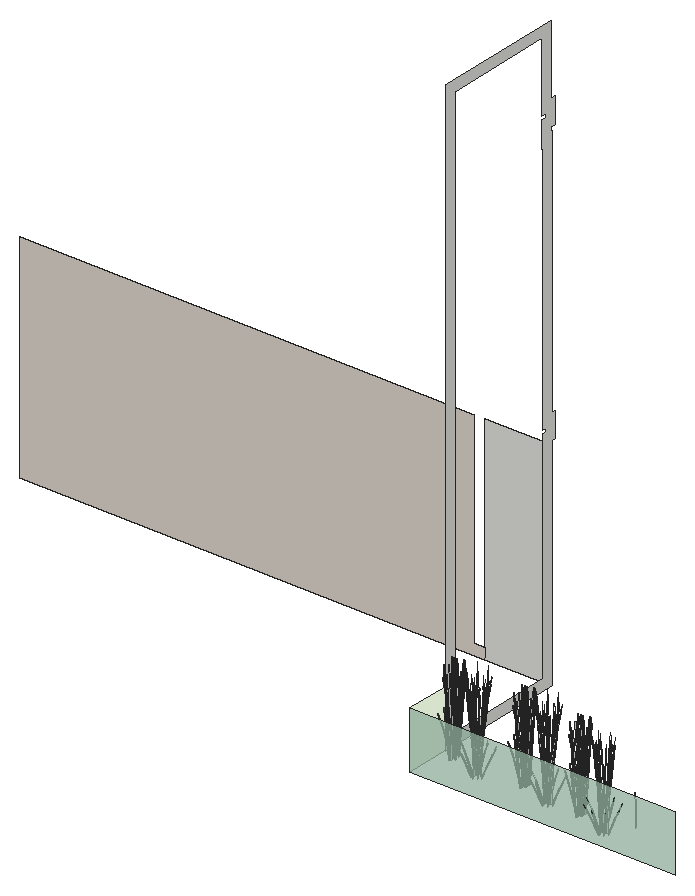
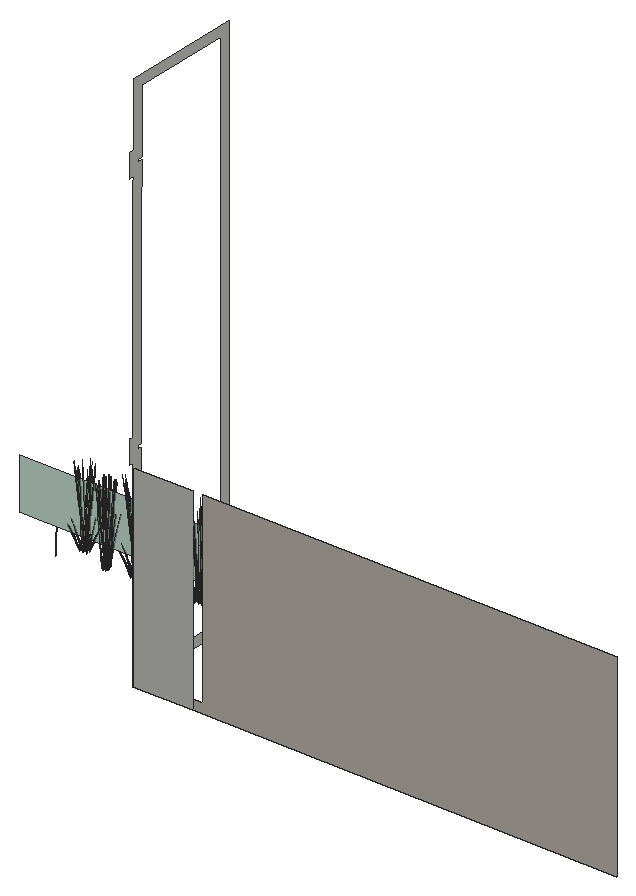
# SketchUp Ruby script. Lengths in inches.
U = 1.inch
M = Sketchup.active_model
def pt(a) = Geom::Point3d.new(a.map { |v| v * U })
def face(e, loops, mat)
  f = e.add_face(loops[0].map { |a| pt(a) })
  loops[1..].each { |l| e.add_face(l.map { |a| pt(a) }).erase! }
  f.material = f.back_material = mat if mat
  f
end
# faces: each face lists its corners as indices into pts; further lists are holes
def faces(e, pts, list, mat = nil) = list.each { |f| face(e, (f[0].is_a?(Array) ? f : [f]).map { |l| l.map { |i| pts[i] } }, mat) }
# xy, xz, yz: faces in a plane at the given z, y or x. An outline is a flat list of corners, or four numbers for a rectangle; further outlines are holes
def ring(l) = l.size == 4 ? [[l[0], l[1]], [l[2], l[1]], [l[2], l[3]], [l[0], l[3]]] : l.each_slice(2).to_a
def flat(e, list, mat, &to3) = list.each { |f| face(e, (f[0].is_a?(Array) ? f : [f]).map { |l| ring(l).map { |u, v| to3.(u, v) } }, mat) }
def xy(e, z, list, mat = nil) = flat(e, list, mat) { |x, y| [x, y, z] }
def xz(e, y, list, mat = nil) = flat(e, list, mat) { |x, z| [x, y, z] }
def yz(e, x, list, mat = nil) = flat(e, list, mat) { |y, z| [x, y, z] }
def lines(e, pts, list) = list.each { |a, b| e.add_line(pt(pts[a]), pt(pts[b])) }
# prism: a flat outline (further loops are holes) pulled along v
def prism(e, loops, v, mat = nil)
  f = face(e, loops, mat); d = Geom::Vector3d.new(v.map { |x| x * U })
  f.pushpull(f.normal.samedirection?(d) ? d.length : -d.length)
end
def box(e, o, s, mat = nil) = prism(e, [[o, [o[0] + s[0], o[1], o[2]], [o[0] + s[0], o[1] + s[1], o[2]], [o[0], o[1] + s[1], o[2]]]], [0, 0, s[2]], mat)
def at(x, y, z, deg = 0) = Geom::Transformation.translation(pt([x, y, z])) * Geom::Transformation.rotation(ORIGIN, Z_AXIS, deg.degrees)
def axes(o, x, y, z) = Geom::Transformation.new([*x, 0, *y, 0, *z, 0, *pt(o).to_a, 1])
def part(name) = M.definitions.add(name)
# library, detail: a bought-in or finely detailed component or shape, given as its bounding box
def library(name, o, s) = part(name).tap { |d| box(d.entities, o, s) }
def detail(e, o, s) = box(e.add_group.entities, o, s)
def put(e, d, t, mat = nil) = e.add_instance(d, t).tap { |i| i.material = mat if mat }
def group(e, t, mat = nil) = e.add_group.tap { |g| g.transformation = t; g.material = mat if mat }.entities
root = M.entities
M.materials.add("Glass_Basic_01").color = [128, 186, 71]
M.materials["Glass_Basic_01"].alpha = 0.25
M.materials.add("LightPink_Translucent").color = [175, 214, 192]
M.materials["LightPink_Translucent"].alpha = 0.75
M.materials.add("ThomThom - Complexion1").color = [221, 214, 204]
c1 = part("blade")
p = [[2.15,0.21,22],[0,0.17,0],[0.09,0.45,0],[2.18,0.31,22],[2.29,0.31,22],[0.38,0.45,0],
  [2.48,0.24,33],[2.49,0.24,33],[2.48,0.22,33]]
faces(c1.entities,p,[[0,1,2,3],[4,5,2,3],[6,3,4,7],[8,0,3,6]])
c2 = part("blade with seeds\#1")
put(c2.entities,c1,at(0,0,0))
c3 = part("seeds")
p = [[0.3,-0.1,1.38],[-0.01,-0.03,1.59],[-0.01,-0.03,0.03],[0.14,-0.07,-0.07],[0.29,-0.03,3],[0.15,0.01,3.11]]
faces(c3.entities,p,[[0,1,2,3],[1,0,4,5]],"LightPink_Translucent")
c4 = part("blade with seeds")
put(c4.entities,c1,at(0,0,0))
put(c4.entities,c3,axes([2.4,0.25,30.99],[1.5799,-0.05474,1.17369],[-0.12525,1.92788,0.29478],[-0.07173,-0.02425,1.56792]))
xz(root,222,[[366,138,510,169.19]],"LightPink_Translucent")
xz(root,318,[[330,138,366,255]])
xz(root,318,[[77.51,138,77.51,255,324,255,324,144,330,144,330,138]],"ThomThom - Complexion1")
yz(root,366,[[[246,138,318,138,318,257,320,257,320,271,318,271,318,408,317.22,408,317.22,410,320,410,320,424,317.22,424,317.22,462,246,462],[252,144,252,456,311.22,456,311.22,418,314,418,314,416,311.22,416,311.22,402,312,402,312,265,314,265,314,263,312,263,312,144]]])
yz(root,366,[[222,138,246,169.19]],"Glass_Basic_01")
put(root,c2,axes([371.2,243.44,138.46],[0.2186,0.34354,-0.03193],[-0.23941,0.31478,-0.14479],[-0.06784,0.02216,0.47756]))
put(root,c2,axes([371.66,244.125,138.66],[-0.38183,0.31082,0],[-0.21294,-0.52,-0.42336],[-0.0485,-0.11843,1.343]))
put(root,c2,axes([371.6,245.15,138.46],[0.31114,0.14341,-0.03193],[-0.09571,0.44138,-0.14479],[-0.05089,0.06702,0.47756]))
put(root,c2,axes([372.72,243.51,138.91],[-0.43479,0.05793,-0.23868],[-0.02629,-0.60335,-0.41019],[-0.05792,-0.10625,1.31016]))
put(root,c2,axes([373.17,243.79,138.91],[-0.18181,0.55986,-0.23868],[-0.38374,-0.26958,-0.41019],[-0.09422,0.01759,1.31016]))
put(root,c2,axes([373.02,245.39,138.66],[0,0.62163,0],[-0.42587,0,-0.42336],[-0.097,0,1.343]))
put(root,c2,axes([372.91,244.91,138.63],[0.32036,0.46241,0.25231],[-0.31699,0.46269,-0.29936],[-0.09098,0.01615,1.35263]))
put(root,c2,axes([373.57,243.65,138.72],[-0.45152,-0.13176,-0.1922],[0.07871,-0.62475,0.4206],[-0.06235,0.10917,1.28336]))
put(root,c2,axes([371.76,241.84,138.67],[-0.38183,-0.31082,0],[0.21294,-0.52,-0.42336],[0.0485,-0.11843,1.343]))
put(root,c2,axes([373.27,240.61,138.34],[0.04573,0.32019,1.16148],[-0.36399,0.05096,0.06648],[-0.05509,-0.22426,0.66092]))
put(root,c2,axes([372.94,240.03,138.57],[-0.24366,0.30821,-0.05322],[-0.22326,-0.33756,-0.24131],[-0.01572,-0.09565,0.79594]))
put(root,c2,axes([372.98,242.86,138.53],[-0.4409,0,0],[0,-0.62163,0],[0,0,1.47217]))
put(root,c2,axes([372.43,244.08,138.02],[0.15256,0.48933,1.05766],[-0.43772,0.15575,0.41096],[0.00728,-0.30048,1.20297]))
put(root,c2,axes([373.32,242.7,138.6],[-0.32797,0.46241,-0.0503],[-0.32817,-0.46269,0],[-0.01145,0.01615,1.4403]))
put(root,c2,axes([372.66,242.82,138.91],[-0.25298,-0.50193,-0.23868],[0.35745,-0.33378,-0.41019],[0.0363,-0.12384,1.31016]))
put(root,c2,axes([373.57,243.38,138.91],[0.25298,0.50193,-0.23868],[-0.35745,0.33378,-0.41019],[-0.0363,0.12384,1.31016]))
put(root,c2,axes([373.07,242.44,138.53],[0,-0.5562,0],[0.39449,0,0],[0,0,1.46356]))
put(root,c2,axes([373.99,243.12,138.53],[-0.32851,0.1622,0],[-0.11504,-0.46318,0],[0,0,1.26638]))
put(root,c2,axes([373.24,242.45,138.53],[0.24613,-0.34702,0],[0.24613,0.34702,0],[0,0,1.38858]))
put(root,c2,axes([373.95,242.51,138.51],[-0.12929,-0.52192,-0.15749],[0.37242,-0.1834,0.00007],[-0.01429,-0.05761,1.42656]))
put(root,c2,axes([373.6875,242.8125,138.74],[-0.30669,0.48544,-0.20666],[-0.34439,-0.40848,0.45226],[0.03588,0.13072,1.37996]))
put(root,c2,axes([374.14,243.23,138.52],[-0.17107,0.50118,0],[-0.35546,-0.2412,0],[0,0,1.33477]))
put(root,c2,axes([373.15,242.54,138.6],[0.44068,0,-0.04624],[0,0.62163,0],[0.01385,0,1.47144]))
put(root,c2,axes([374.47,244.36,138.66],[0.38183,0.31082,0],[-0.21294,0.52,-0.42336],[-0.0485,0.11843,1.343]))
put(root,c2,axes([374.15,242.66,138.53],[0.17107,-0.50118,0],[0.35546,0.2412,0],[0,0,1.43523]))
put(root,c2,axes([374.53,242.46,138.52],[-0.38316,0.30694,-0.04218],[-0.21294,-0.52,0.42336],[0.03648,0.12814,1.34234]))
put(root,c2,axes([374,242.84,138.6],[0.43775,-0.21614,-0.04932],[0.15339,0.61757,0],[0.01529,-0.00755,1.41242]))
put(root,c2,axes([373.43,241.06,138.52],[-0.00305,0.62132,-0.04082],[-0.42587,0,0.4097],[0.09695,0.01953,1.29904]))
put(root,c2,axes([373.21,240.81,138.67],[0,-0.62163,0],[0.42587,0,-0.42336],[0.097,0,1.343]))
put(root,c2,axes([373.06,242.4,138.91],[0.18181,-0.55986,-0.23868],[0.38374,0.26958,-0.41019],[0.09422,-0.01759,1.31016]))
put(root,c2,axes([373.52,242.68,138.91],[0.43479,-0.05793,-0.23868],[0.02629,0.60335,-0.41019],[0.05792,0.10625,1.31016]))
put(root,c2,axes([374.33,242.45,138.63],[0.12385,-0.62237,0.25231],[0.4427,0.1557,-0.29936],[0.05541,0.10301,1.35263]))
put(root,c2,axes([374.57,242.07,138.66],[0.38183,-0.31082,0],[0.21294,0.52,-0.42336],[0.0485,0.11843,1.343]))
put(root,c4,axes([388.53,236.22,138.53],[0.01212,0.07018,1.60472],[-0.24435,0.36652,-0.24515],[-0.17356,-0.01847,0.27334]))
put(root,c4,axes([388.4,238.1875,138.53],[0.06411,0.04449,1.60472],[0.1087,0.41223,-0.24515],[-0.14209,0.08791,0.27334]))
put(root,c4,axes([389.28,234.4,138.53],[-0.0463,0.05867,1.60472],[-0.46786,0.12648,-0.24515],[-0.11302,-0.11506,0.27334]))
put(root,c4,axes([390.69,236.93,139.6],[-0.48255,0.29566,-0.26477],[-0.32089,-0.41776,-0.45502],[-0.11906,-0.04243,1.45334]))
put(root,c4,axes([389.6,237.55,139.02],[-0.11227,-0.38804,-0.2819],[0.44589,-0.11019,0.2819],[-0.08989,-0.04475,1.26466]))
put(root,c4,axes([390.39,236.72,139.18],[-0.28711,-0.37379,-0.40713],[0.43489,-0.26322,0.19594],[-0.09291,-0.04625,1.30716]))
put(root,c4,axes([391,236.98,139.18],[-0.519,0.02749,-0.40713],[-0.04694,-0.45634,0.19594],[-0.09291,0.04625,1.30716]))
put(root,c4,axes([391.4375,237.99,139.02],[-0.44589,-0.11019,-0.2819],[0.11227,-0.38804,0.2819],[-0.08989,0.04475,1.26466]))
put(root,c4,axes([390.29,236.46,139.6],[-0.53825,-0.21249,-0.26477],[0.25917,-0.44849,-0.45502],[-0.01692,-0.11011,1.45334]))
put(root,c4,axes([391.36,236.86,139.6],[0.05569,0.50815,-0.26477],[-0.58006,0.03072,-0.45502],[-0.10214,0.06769,1.45334]))
put(root,c4,axes([389.125,235.95,139.02],[0.33362,-0.27785,-0.2819],[0.33362,0.27785,0.2819],[0,-0.08949,1.26466]))
put(root,c4,axes([390.71,233.84,138.53],[-0.08017,0.01605,1.60472],[-0.44332,-0.18061,-0.24515],[0.00744,-0.15065,0.27334]))
put(root,c4,axes([390.35,236.125,139.18],[0.23189,-0.40128,-0.40713],[0.48183,0.19312,0.19594],[0,-0.0925,1.30716]))
put(root,c4,axes([390.38,238.23,138.53],[0.07735,-0.02423,1.60472],[0.46528,0.13338,-0.24515],[0.01361,0.15033,0.27334]))
put(root,c4,axes([391.57,236.66,139.18],[-0.23189,0.40128,-0.40713],[-0.48183,-0.19312,0.19594],[0,0.0925,1.30716]))
put(root,c4,axes([392.8,236.83,139.02],[-0.33362,0.27785,-0.2819],[-0.33362,-0.27785,0.2819],[0,0.08949,1.26466]))
put(root,c4,axes([390.5625,235.93,139.6],[-0.05569,-0.50815,-0.26477],[0.58006,-0.03072,-0.45502],[0.10214,-0.06769,1.45334]))
put(root,c4,axes([391.63,236.33,139.6],[0.53825,0.21249,-0.26477],[-0.25917,0.44849,-0.45502],[0.01692,0.11011,1.45334]))
put(root,c4,axes([390.49,234.8,139.02],[0.44589,0.11019,-0.2819],[-0.11227,0.38804,0.2819],[0.08989,-0.04475,1.26466]))
put(root,c4,axes([391.54,236.07,139.18],[0.28711,0.37379,-0.40713],[-0.43489,0.26322,0.19594],[0.09291,0.04625,1.30716]))
put(root,c4,axes([392.32,235.24,139.02],[0.11227,0.38804,-0.2819],[-0.44589,0.11019,0.2819],[0.08989,0.04475,1.26466]))
put(root,c4,axes([391.23,235.86,139.6],[0.48255,-0.29566,-0.26477],[0.32089,0.41776,-0.45502],[0.11906,0.04243,1.45334]))
put(root,c4,axes([390.01,235.6,138.62],[-0.47044,0.17829,1.17325],[-0.14973,-0.51157,0.45588],[0.28888,0.00851,1.33444]))
put(root,c4,axes([392.68,234.61,138.53],[-0.07154,-0.03508,1.60472],[-0.18375,-0.39195,-0.24515],[0.12396,-0.10636,0.27334]))
put(root,c4,axes([392.43,238.24,138.53],[0.03482,-0.06429,1.60472],[0.43839,-0.18935,-0.24515],[0.13291,0.098,0.27334]))
put(root,c4,axes([393.6875,236.29,138.53],[-0.02498,-0.06761,1.60472],[0.17324,-0.39549,-0.24515],[0.17476,-0.00569,0.27334]))
put(root,c2,axes([409.4,243.44,138.46],[0.2186,0.34354,-0.03193],[-0.23941,0.31478,-0.14479],[-0.06784,0.02216,0.47756]))
put(root,c2,axes([409.86,244.125,138.66],[-0.38183,0.31082,0],[-0.21294,-0.52,-0.42336],[-0.0485,-0.11843,1.343]))
put(root,c2,axes([409.79,245.15,138.46],[0.31114,0.14341,-0.03193],[-0.09571,0.44138,-0.14479],[-0.05089,0.06702,0.47756]))
put(root,c2,axes([410.91,243.51,138.91],[-0.43479,0.05793,-0.23868],[-0.02629,-0.60335,-0.41019],[-0.05792,-0.10625,1.31016]))
put(root,c2,axes([411.37,243.79,138.91],[-0.18181,0.55986,-0.23868],[-0.38374,-0.26958,-0.41019],[-0.09422,0.01759,1.31016]))
put(root,c2,axes([411.21,245.39,138.66],[0,0.62163,0],[-0.42587,0,-0.42336],[-0.097,0,1.343]))
put(root,c2,axes([411.1,244.91,138.63],[0.32036,0.46241,0.25231],[-0.31699,0.46269,-0.29936],[-0.09098,0.01615,1.35263]))
put(root,c2,axes([411.77,243.65,138.72],[-0.45152,-0.13176,-0.1922],[0.07871,-0.62475,0.4206],[-0.06235,0.10917,1.28336]))
put(root,c2,axes([409.95,241.84,138.67],[-0.38183,-0.31082,0],[0.21294,-0.52,-0.42336],[0.0485,-0.11843,1.343]))
put(root,c2,axes([411.46,240.61,138.34],[0.04573,0.32019,1.16148],[-0.36399,0.05096,0.06648],[-0.05509,-0.22426,0.66092]))
put(root,c2,axes([411.14,240.03,138.57],[-0.24366,0.30821,-0.05322],[-0.22326,-0.33756,-0.24131],[-0.01572,-0.09565,0.79594]))
put(root,c2,axes([411.17,242.86,138.53],[-0.4409,0,0],[0,-0.62163,0],[0,0,1.47217]))
put(root,c2,axes([410.63,244.08,138.02],[0.15256,0.48933,1.05766],[-0.43772,0.15575,0.41096],[0.00728,-0.30048,1.20297]))
put(root,c2,axes([411.51,242.7,138.6],[-0.32797,0.46241,-0.0503],[-0.32817,-0.46269,0],[-0.01145,0.01615,1.4403]))
put(root,c2,axes([410.85,242.82,138.91],[-0.25298,-0.50193,-0.23868],[0.35745,-0.33378,-0.41019],[0.0363,-0.12384,1.31016]))
put(root,c2,axes([411.77,243.38,138.91],[0.25298,0.50193,-0.23868],[-0.35745,0.33378,-0.41019],[-0.0363,0.12384,1.31016]))
put(root,c2,axes([411.27,242.44,138.53],[0,-0.5562,0],[0.39449,0,0],[0,0,1.46356]))
put(root,c2,axes([412.1875,243.12,138.53],[-0.32851,0.1622,0],[-0.11504,-0.46318,0],[0,0,1.26638]))
put(root,c2,axes([411.4375,242.45,138.53],[0.24613,-0.34702,0],[0.24613,0.34702,0],[0,0,1.38858]))
put(root,c2,axes([412.14,242.51,138.51],[-0.12929,-0.52192,-0.15749],[0.37242,-0.1834,0.00007],[-0.01429,-0.05761,1.42656]))
put(root,c2,axes([411.88,242.8125,138.74],[-0.30669,0.48544,-0.20666],[-0.34439,-0.40848,0.45226],[0.03588,0.13072,1.37996]))
put(root,c2,axes([412.34,243.23,138.52],[-0.17107,0.50118,0],[-0.35546,-0.2412,0],[0,0,1.33477]))
put(root,c2,axes([411.35,242.54,138.6],[0.44068,0,-0.04624],[0,0.62163,0],[0.01385,0,1.47144]))
put(root,c2,axes([412.67,244.36,138.66],[0.38183,0.31082,0],[-0.21294,0.52,-0.42336],[-0.0485,0.11843,1.343]))
put(root,c2,axes([412.34,242.66,138.53],[0.17107,-0.50118,0],[0.35546,0.2412,0],[0,0,1.43523]))
put(root,c2,axes([412.72,242.46,138.52],[-0.38316,0.30694,-0.04218],[-0.21294,-0.52,0.42336],[0.03648,0.12814,1.34234]))
put(root,c2,axes([412.2,242.84,138.6],[0.43775,-0.21614,-0.04932],[0.15339,0.61757,0],[0.01529,-0.00755,1.41242]))
put(root,c2,axes([411.625,241.06,138.52],[-0.00305,0.62132,-0.04082],[-0.42587,0,0.4097],[0.09695,0.01953,1.29904]))
put(root,c2,axes([411.41,240.81,138.67],[0,-0.62163,0],[0.42587,0,-0.42336],[0.097,0,1.343]))
put(root,c2,axes([411.25,242.4,138.91],[0.18181,-0.55986,-0.23868],[0.38374,0.26958,-0.41019],[0.09422,-0.01759,1.31016]))
put(root,c2,axes([411.71,242.68,138.91],[0.43479,-0.05793,-0.23868],[0.02629,0.60335,-0.41019],[0.05792,0.10625,1.31016]))
put(root,c2,axes([412.52,242.45,138.63],[0.12385,-0.62237,0.25231],[0.4427,0.1557,-0.29936],[0.05541,0.10301,1.35263]))
put(root,c2,axes([412.76,242.07,138.66],[0.38183,-0.31082,0],[0.21294,0.52,-0.42336],[0.0485,0.11843,1.343]))
put(root,c4,axes([426.73,236.22,138.53],[0.01212,0.07018,1.60472],[-0.24435,0.36652,-0.24515],[-0.17356,-0.01847,0.27334]))
put(root,c4,axes([426.59,238.1875,138.53],[0.06411,0.04449,1.60472],[0.1087,0.41223,-0.24515],[-0.14209,0.08791,0.27334]))
put(root,c4,axes([427.47,234.4,138.53],[-0.0463,0.05867,1.60472],[-0.46786,0.12648,-0.24515],[-0.11302,-0.11506,0.27334]))
put(root,c4,axes([428.89,236.93,139.6],[-0.48255,0.29566,-0.26477],[-0.32089,-0.41776,-0.45502],[-0.11906,-0.04243,1.45334]))
put(root,c4,axes([427.8,237.55,139.02],[-0.11227,-0.38804,-0.2819],[0.44589,-0.11019,0.2819],[-0.08989,-0.04475,1.26466]))
put(root,c4,axes([428.58,236.72,139.18],[-0.28711,-0.37379,-0.40713],[0.43489,-0.26322,0.19594],[-0.09291,-0.04625,1.30716]))
put(root,c4,axes([429.19,236.98,139.18],[-0.519,0.02749,-0.40713],[-0.04694,-0.45634,0.19594],[-0.09291,0.04625,1.30716]))
put(root,c4,axes([429.63,237.99,139.02],[-0.44589,-0.11019,-0.2819],[0.11227,-0.38804,0.2819],[-0.08989,0.04475,1.26466]))
put(root,c4,axes([428.49,236.46,139.6],[-0.53825,-0.21249,-0.26477],[0.25917,-0.44849,-0.45502],[-0.01692,-0.11011,1.45334]))
put(root,c4,axes([429.56,236.86,139.6],[0.05569,0.50815,-0.26477],[-0.58006,0.03072,-0.45502],[-0.10214,0.06769,1.45334]))
put(root,c4,axes([427.32,235.95,139.02],[0.33362,-0.27785,-0.2819],[0.33362,0.27785,0.2819],[0,-0.08949,1.26466]))
put(root,c4,axes([428.91,233.84,138.53],[-0.08017,0.01605,1.60472],[-0.44332,-0.18061,-0.24515],[0.00744,-0.15065,0.27334]))
put(root,c4,axes([428.55,236.125,139.18],[0.23189,-0.40128,-0.40713],[0.48183,0.19312,0.19594],[0,-0.0925,1.30716]))
put(root,c4,axes([428.57,238.23,138.53],[0.07735,-0.02423,1.60472],[0.46528,0.13338,-0.24515],[0.01361,0.15033,0.27334]))
put(root,c4,axes([429.77,236.66,139.18],[-0.23189,0.40128,-0.40713],[-0.48183,-0.19312,0.19594],[0,0.0925,1.30716]))
put(root,c4,axes([430.99,236.83,139.02],[-0.33362,0.27785,-0.2819],[-0.33362,-0.27785,0.2819],[0,0.08949,1.26466]))
put(root,c4,axes([428.76,235.93,139.6],[-0.05569,-0.50815,-0.26477],[0.58006,-0.03072,-0.45502],[0.10214,-0.06769,1.45334]))
put(root,c4,axes([429.83,236.33,139.6],[0.53825,0.21249,-0.26477],[-0.25917,0.44849,-0.45502],[0.01692,0.11011,1.45334]))
put(root,c4,axes([428.68,234.8,139.02],[0.44589,0.11019,-0.2819],[-0.11227,0.38804,0.2819],[0.08989,-0.04475,1.26466]))
put(root,c4,axes([429.73,236.07,139.18],[0.28711,0.37379,-0.40713],[-0.43489,0.26322,0.19594],[0.09291,0.04625,1.30716]))
put(root,c4,axes([430.52,235.24,139.02],[0.11227,0.38804,-0.2819],[-0.44589,0.11019,0.2819],[0.08989,0.04475,1.26466]))
put(root,c4,axes([429.43,235.86,139.6],[0.48255,-0.29566,-0.26477],[0.32089,0.41776,-0.45502],[0.11906,0.04243,1.45334]))
put(root,c4,axes([428.21,235.6,138.62],[-0.47044,0.17829,1.17325],[-0.14973,-0.51157,0.45588],[0.28888,0.00851,1.33444]))
put(root,c4,axes([430.87,234.61,138.53],[-0.07154,-0.03508,1.60472],[-0.18375,-0.39195,-0.24515],[0.12396,-0.10636,0.27334]))
put(root,c4,axes([430.62,238.24,138.53],[0.03482,-0.06429,1.60472],[0.43839,-0.18935,-0.24515],[0.13291,0.098,0.27334]))
put(root,c4,axes([431.88,236.29,138.53],[-0.02498,-0.06761,1.60472],[0.17324,-0.39549,-0.24515],[0.17476,-0.00569,0.27334]))
put(root,c2,axes([443.68,238.625,138.56],[0.2186,0.34354,-0.03193],[-0.23941,0.31478,-0.14479],[-0.06784,0.02216,0.47756]))
put(root,c2,axes([444.14,239.31,138.76],[-0.38183,0.31082,0],[-0.21294,-0.52,-0.42336],[-0.0485,-0.11843,1.343]))
put(root,c2,axes([444.08,240.33,138.56],[0.31114,0.14341,-0.03193],[-0.09571,0.44138,-0.14479],[-0.05089,0.06702,0.47756]))
put(root,c2,axes([445.2,238.7,139],[-0.43479,0.05793,-0.23868],[-0.02629,-0.60335,-0.41019],[-0.05792,-0.10625,1.31016]))
put(root,c2,axes([445.65,238.98,139],[-0.18181,0.55986,-0.23868],[-0.38374,-0.26958,-0.41019],[-0.09422,0.01759,1.31016]))
put(root,c2,axes([445.5,240.57,138.76],[0,0.62163,0],[-0.42587,0,-0.42336],[-0.097,0,1.343]))
put(root,c2,axes([445.39,240.09,138.72],[0.32036,0.46241,0.25231],[-0.31699,0.46269,-0.29936],[-0.09098,0.01615,1.35263]))
put(root,c2,axes([446.06,238.84,138.8125],[-0.45152,-0.13176,-0.1922],[0.07871,-0.62475,0.4206],[-0.06235,0.10917,1.28336]))
put(root,c2,axes([444.24,237.02,138.76],[-0.38183,-0.31082,0],[0.21294,-0.52,-0.42336],[0.0485,-0.11843,1.343]))
put(root,c2,axes([445.75,235.79,138.4375],[0.04573,0.32019,1.16148],[-0.36399,0.05096,0.06648],[-0.05509,-0.22426,0.66092]))
put(root,c2,axes([445.43,235.21,138.67],[-0.24366,0.30821,-0.05322],[-0.22326,-0.33756,-0.24131],[-0.01572,-0.09565,0.79594]))
put(root,c2,axes([445.46,238.04,138.62],[-0.4409,0,0],[0,-0.62163,0],[0,0,1.47217]))
put(root,c2,axes([444.92,239.27,138.12],[0.15256,0.48933,1.05766],[-0.43772,0.15575,0.41096],[0.00728,-0.30048,1.20297]))
put(root,c2,axes([445.8,237.88,138.7],[-0.32797,0.46241,-0.0503],[-0.32817,-0.46269,0],[-0.01145,0.01615,1.4403]))
put(root,c2,axes([445.14,238,139],[-0.25298,-0.50193,-0.23868],[0.35745,-0.33378,-0.41019],[0.0363,-0.12384,1.31016]))
put(root,c2,axes([446.05,238.56,139],[0.25298,0.50193,-0.23868],[-0.35745,0.33378,-0.41019],[-0.0363,0.12384,1.31016]))
put(root,c2,axes([445.56,237.62,138.62],[0,-0.5562,0],[0.39449,0,0],[0,0,1.46356]))
put(root,c2,axes([446.48,238.3,138.62],[-0.32851,0.1622,0],[-0.11504,-0.46318,0],[0,0,1.26638]))
put(root,c2,axes([446.43,237.69,138.61],[-0.12929,-0.52192,-0.15749],[0.37242,-0.1834,0.00007],[-0.01429,-0.05761,1.42656]))
put(root,c2,axes([446.17,238,138.84],[-0.30669,0.48544,-0.20666],[-0.34439,-0.40848,0.45226],[0.03588,0.13072,1.37996]))
put(root,c2,axes([446.625,238.41,138.61],[-0.17107,0.50118,0],[-0.35546,-0.2412,0],[0,0,1.33477]))
put(root,c2,axes([445.63,237.73,138.69],[0.44068,0,-0.04624],[0,0.62163,0],[0.01385,0,1.47144]))
put(root,c2,axes([446.96,239.54,138.76],[0.38183,0.31082,0],[-0.21294,0.52,-0.42336],[-0.0485,0.11843,1.343]))
put(root,c2,axes([446.63,237.84,138.62],[0.17107,-0.50118,0],[0.35546,0.2412,0],[0,0,1.43523]))
put(root,c2,axes([447.01,237.64,138.61],[-0.38316,0.30694,-0.04218],[-0.21294,-0.52,0.42336],[0.03648,0.12814,1.34234]))
put(root,c2,axes([446.49,238.02,138.69],[0.43775,-0.21614,-0.04932],[0.15339,0.61757,0],[0.01529,-0.00755,1.41242]))
put(root,c2,axes([445.91,236.24,138.62],[-0.00305,0.62132,-0.04082],[-0.42587,0,0.4097],[0.09695,0.01953,1.29904]))
put(root,c2,axes([445.69,235.99,138.76],[0,-0.62163,0],[0.42587,0,-0.42336],[0.097,0,1.343]))
put(root,c2,axes([445.54,237.58,139],[0.18181,-0.55986,-0.23868],[0.38374,0.26958,-0.41019],[0.09422,-0.01759,1.31016]))
put(root,c2,axes([446,237.86,139],[0.43479,-0.05793,-0.23868],[0.02629,0.60335,-0.41019],[0.05792,0.10625,1.31016]))
put(root,c2,axes([446.8125,237.63,138.72],[0.12385,-0.62237,0.25231],[0.4427,0.1557,-0.29936],[0.05541,0.10301,1.35263]))
put(root,c2,axes([447.05,237.25,138.76],[0.38183,-0.31082,0],[0.21294,0.52,-0.42336],[0.0485,0.11843,1.343]))
put(root,c4,axes([461.01,231.41,138.625],[0.01212,0.07018,1.60472],[-0.24435,0.36652,-0.24515],[-0.17356,-0.01847,0.27334]))
put(root,c4,axes([460.88,233.37,138.625],[0.06411,0.04449,1.60472],[0.1087,0.41223,-0.24515],[-0.14209,0.08791,0.27334]))
put(root,c4,axes([461.76,229.58,138.625],[-0.0463,0.05867,1.60472],[-0.46786,0.12648,-0.24515],[-0.11302,-0.11506,0.27334]))
put(root,c4,axes([462.08,232.73,139.11],[-0.11227,-0.38804,-0.2819],[0.44589,-0.11019,0.2819],[-0.08989,-0.04475,1.26466]))
put(root,c4,axes([462.87,231.9,139.28],[-0.28711,-0.37379,-0.40713],[0.43489,-0.26322,0.19594],[-0.09291,-0.04625,1.30716]))
put(root,c4,axes([463.48,232.17,139.28],[-0.519,0.02749,-0.40713],[-0.04694,-0.45634,0.19594],[-0.09291,0.04625,1.30716]))
put(root,c4,axes([463.92,233.17,139.11],[-0.44589,-0.11019,-0.2819],[0.11227,-0.38804,0.2819],[-0.08989,0.04475,1.26466]))
put(root,c4,axes([461.61,231.14,139.11],[0.33362,-0.27785,-0.2819],[0.33362,0.27785,0.2819],[0,-0.08949,1.26466]))
put(root,c4,axes([463.2,229.03,138.625],[-0.08017,0.01605,1.60472],[-0.44332,-0.18061,-0.24515],[0.00744,-0.15065,0.27334]))
put(root,c4,axes([462.83,231.31,139.28],[0.23189,-0.40128,-0.40713],[0.48183,0.19312,0.19594],[0,-0.0925,1.30716]))
put(root,c4,axes([462.86,233.41,138.625],[0.07735,-0.02423,1.60472],[0.46528,0.13338,-0.24515],[0.01361,0.15033,0.27334]))
put(root,c4,axes([464.06,231.84,139.28],[-0.23189,0.40128,-0.40713],[-0.48183,-0.19312,0.19594],[0,0.0925,1.30716]))
put(root,c4,axes([465.28,232.02,139.11],[-0.33362,0.27785,-0.2819],[-0.33362,-0.27785,0.2819],[0,0.08949,1.26466]))
put(root,c4,axes([462.97,229.98,139.11],[0.44589,0.11019,-0.2819],[-0.11227,0.38804,0.2819],[0.08989,-0.04475,1.26466]))
put(root,c4,axes([464.02,231.25,139.28],[0.28711,0.37379,-0.40713],[-0.43489,0.26322,0.19594],[0.09291,0.04625,1.30716]))
put(root,c4,axes([464.81,230.42,139.11],[0.11227,0.38804,-0.2819],[-0.44589,0.11019,0.2819],[0.08989,0.04475,1.26466]))
put(root,c4,axes([465.16,229.79,138.625],[-0.07154,-0.03508,1.60472],[-0.18375,-0.39195,-0.24515],[0.12396,-0.10636,0.27334]))
put(root,c4,axes([464.91,233.43,138.625],[0.03482,-0.06429,1.60472],[0.43839,-0.18935,-0.24515],[0.13291,0.098,0.27334]))
put(root,c4,axes([466.17,231.47,138.625],[-0.02498,-0.06761,1.60472],[0.17324,-0.39549,-0.24515],[0.17476,-0.00569,0.27334]))
put(root,c2,axes([471.41,243.44,138.46],[0.2186,0.34354,-0.03193],[-0.23941,0.31478,-0.14479],[-0.06784,0.02216,0.47756]))
